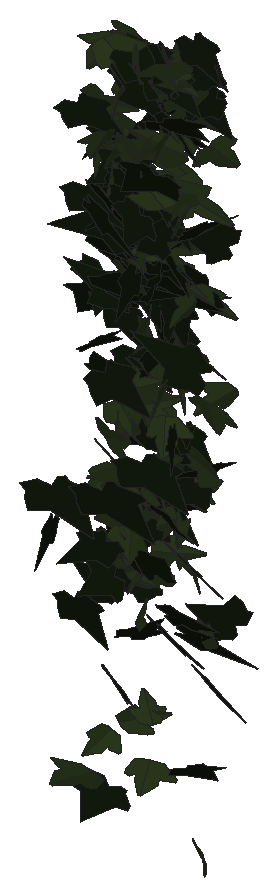
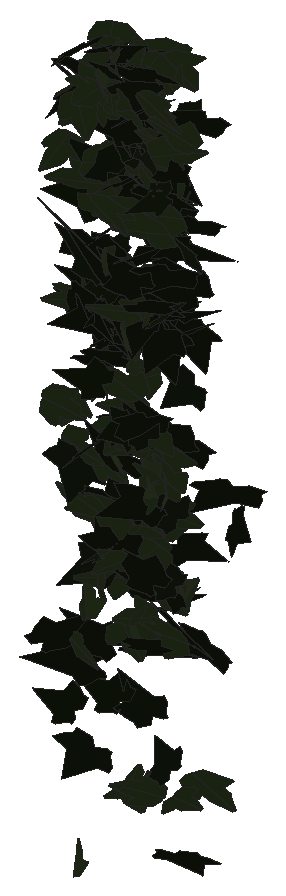
# SketchUp Ruby script. Lengths in millimetres.
U = 1.mm
M = Sketchup.active_model
def pt(a) = Geom::Point3d.new(a.map { |v| v * U })
def face(e, loops, mat)
  f = e.add_face(loops[0].map { |a| pt(a) })
  loops[1..].each { |l| e.add_face(l.map { |a| pt(a) }).erase! }
  f.material = f.back_material = mat if mat
  f
end
# faces: each face lists its corners as indices into pts; further lists are holes
def faces(e, pts, list, mat = nil) = list.each { |f| face(e, (f[0].is_a?(Array) ? f : [f]).map { |l| l.map { |i| pts[i] } }, mat) }
# xy, xz, yz: faces in a plane at the given z, y or x. An outline is a flat list of corners, or four numbers for a rectangle; further outlines are holes
def ring(l) = l.size == 4 ? [[l[0], l[1]], [l[2], l[1]], [l[2], l[3]], [l[0], l[3]]] : l.each_slice(2).to_a
def flat(e, list, mat, &to3) = list.each { |f| face(e, (f[0].is_a?(Array) ? f : [f]).map { |l| ring(l).map { |u, v| to3.(u, v) } }, mat) }
def xy(e, z, list, mat = nil) = flat(e, list, mat) { |x, y| [x, y, z] }
def xz(e, y, list, mat = nil) = flat(e, list, mat) { |x, z| [x, y, z] }
def yz(e, x, list, mat = nil) = flat(e, list, mat) { |y, z| [x, y, z] }
def lines(e, pts, list) = list.each { |a, b| e.add_line(pt(pts[a]), pt(pts[b])) }
# prism: a flat outline (further loops are holes) pulled along v
def prism(e, loops, v, mat = nil)
  f = face(e, loops, mat); d = Geom::Vector3d.new(v.map { |x| x * U })
  f.pushpull(f.normal.samedirection?(d) ? d.length : -d.length)
end
def box(e, o, s, mat = nil) = prism(e, [[o, [o[0] + s[0], o[1], o[2]], [o[0] + s[0], o[1] + s[1], o[2]], [o[0], o[1] + s[1], o[2]]]], [0, 0, s[2]], mat)
def at(x, y, z, deg = 0) = Geom::Transformation.translation(pt([x, y, z])) * Geom::Transformation.rotation(ORIGIN, Z_AXIS, deg.degrees)
def axes(o, x, y, z) = Geom::Transformation.new([*x, 0, *y, 0, *z, 0, *pt(o).to_a, 1])
def part(name) = M.definitions.add(name)
# library, detail: a bought-in or finely detailed component or shape, given as its bounding box
def library(name, o, s) = part(name).tap { |d| box(d.entities, o, s) }
def detail(e, o, s) = box(e.add_group.entities, o, s)
def put(e, d, t, mat = nil) = e.add_instance(d, t).tap { |i| i.material = mat if mat }
def group(e, t, mat = nil) = e.add_group.tap { |g| g.transformation = t; g.material = mat if mat }.entities
root = M.entities
M.materials.add("efeu1").color = [18, 25, 13]
M.materials.add("efeu2").color = [43, 57, 29]
c1 = part("ivyleaf_9")
p = [[39.1,54.8,31.7],[34.5,51.8,30.2],[-5.3,25.2,17.3],[-17.9,28.3,20.9],[-21.6,21.7,17],[-20.2,4.3,5.3],
  [-22.9,-0.3,2.5],[-17.1,-4,-0.6],[-2,-2.1,-1.2],[-0.7,-15.4,-10.1],[16.6,-22.3,-16.7],[21.1,-15.1,-12.5],
  [32.7,-10.7,-11],[46.1,-1.8,-6.6],[30.8,11.2,3.8]]
faces(c1.entities,p,[[0,1,2,3,4,5,6,7,8,9,10,11,12,13,14]],"efeu1")
c2 = part("ivyleaf_10")
p = [[0,12.8,-0.8],[-1.5,51.3,-10.9],[-4.9,51,-11.6],[-13.6,26.5,-7.3],[-13.2,15.9,-4.6],[-21.1,19.3,-7.2],
  [-29.5,16.3,-8.3],[-29.2,8.3,-6.2],[-19.7,-9.8,0.5],[-7.6,-13,4],[1,-12.2,5.8],[-0.4,51.1,-11.1],
  [-1.5,51.1,-10.9],[1,-12.4,5.9],[16.9,-12.4,3.5],[35.1,9.1,-5.1],[35,12.9,-6.1],[20.5,16.4,-4.9],
  [15.8,15,-3.8],[15.3,27.6,-7.1],[12.8,31.3,-7.8]]
faces(c2.entities,p,[[0,1,2,3,4,5,6,7,8,9,10],[11,12,0,13,14,15,16,17,18,19,20]],"efeu2")
put(root,c1,axes([2946.5,702.1,1430.8],[1.33754,-0.78365,-0.25205],[-0.30578,0.19446,-1.05258],[1.53656,0.72085,0.00994]))
put(root,c1,axes([2949.3,732.1,1125.1],[0.41508,-0.64574,-0.82159],[-0.25105,0.81557,-0.67602],[1.9729,0.23964,0.08683]))
put(root,c1,axes([2822.1,753.9,808],[-0.38061,0.24155,-0.98303],[1.27424,-0.71998,-0.31312],[-1.44495,-0.69854,-0.01719]))
put(root,c1,axes([2935.6,741.6,908.7],[-0.47588,-0.33732,-0.96585],[1.22364,0.72159,-0.41846],[1.51454,-0.68898,0.03461]))
put(root,c1,axes([2823.5,757.3,870.8],[-0.318,-0.64504,-0.79131],[0.5195,0.74442,-0.66445],[1.87224,-0.31611,0.04997]))
put(root,c1,axes([2974.1,780.6,1392.1],[-0.42556,-0.7327,0.45613],[-0.26926,-0.4337,-0.76602],[1.62038,-0.26449,-0.0075]))
put(root,c2,axes([2862.7,783.2,369.6],[-1.05005,-0.34553,0.61966],[-0.9573,-0.3631,-0.65033],[0.95229,-0.74602,0.02952]))
put(root,c1,axes([3000.5,781.7,1472.3],[0.68765,0.27193,-0.7739],[-1.19118,-0.45523,-0.45216],[-1.00913,0.72266,0.00638]))
put(root,c2,axes([3005.8,797.6,1091.6],[0.64746,-0.69061,0.64263],[0.46311,-0.59578,-0.76908],[1.73463,0.41684,-0.03454]))
put(root,c2,axes([2939.5,791.3,1504],[-0.96338,0.63955,-0.34988],[0.3885,-0.28456,-0.81548],[-1.33192,-0.54559,0.0152]))
put(root,c1,axes([2884.3,804.9,774.7],[-0.06144,-0.00892,-0.90166],[0.09196,-0.90096,0.00718],[-1.71366,-0.04803,0.03271]))
put(root,c2,axes([2883.4,802.4,1492.8],[-0.3913,-0.84361,0.13688],[-0.05405,-0.13396,-0.8683],[1.62566,-0.20752,0.00408]))
put(root,c1,axes([2969.8,796.5,945],[-0.29803,-0.55605,-0.80167],[0.77605,0.70032,-0.5654],[1.68688,-0.42042,0.11847]))
put(root,c1,axes([2941.8,807.7,1262],[-1.14315,0.31014,-0.74291],[1.21653,-0.37977,-0.67534],[-0.93146,-0.87663,0.02973]))
put(root,c2,axes([2917.2,802.9,909.6],[-0.86882,-0.86224,0.07932],[-0.05696,-0.0739,-0.97559],[1.64696,-0.45741,0.0081]))
put(root,c1,axes([2813.5,825.5,638.5],[-0.50737,-0.15268,-0.86245],[1.60954,0.18967,-0.29499],[0.43368,-0.88256,0.08581]))
put(root,c1,axes([2865.4,836.4,1351],[0.31051,-0.48763,0.92572],[0.80832,-0.82538,-0.50963],[1.81988,0.4498,0.06841]))
put(root,c1,axes([3044,831.6,1119.7],[-0.90393,-0.94187,-0.19726],[-0.16554,-0.17706,1.05485],[-1.82397,0.48285,0.00202]))
put(root,c1,axes([2872.5,841.2,694.4],[-0.6415,-0.54818,0.64582],[-0.65457,-0.54665,-0.6435],[1.47335,-0.48154,-0.0047]))
put(root,c1,axes([2828.8,815.6,1522.1],[0.05715,-0.35847,-0.79405],[0.35505,0.77874,-0.3445],[1.61964,-0.15806,0.10354]))
put(root,c2,axes([2971.9,827.2,1397.8],[0.86523,0.63733,0.38042],[-0.42946,-0.30632,0.78284],[1.34575,-0.50751,0.00524]))
put(root,c2,axes([3019.3,830.7,1389.7],[0.47653,-0.88746,0.00656],[0.00339,-0.00631,-0.9221],[1.68905,0.25039,0]))
put(root,c1,axes([2990.6,840.5,988.8],[-0.42942,-0.00366,-0.85863],[1.43073,-0.4298,-0.19572],[-0.7896,-0.7768,0.11233]))
put(root,c1,axes([2987.6,824.9,1333.3],[-1.1226,0.00585,-0.65301],[-1.24283,-0.01087,0.58976],[-0.00789,0.8799,0.01163]))
put(root,c2,axes([2900.3,838.1,806.8],[-1.15154,-0.78668,-0.1797],[-0.20357,-0.14443,0.99244],[-1.52222,0.61443,0.00322]))
put(root,c2,axes([2921.1,820.2,1053.7],[0.00615,-0.05009,-0.94639],[0.88673,0.82421,-0.04203],[1.57067,-0.46512,0.02743]))
put(root,c2,axes([2930.4,845.1,1570.4],[-0.98618,0.08628,0.76506],[1.36089,-0.28793,0.51677],[0.54319,0.87802,0.09429]))
put(root,c1,axes([2964,839.2,1573.9],[-1.49463,-0.31379,-0.39363],[-0.69423,-0.14797,0.84569],[-0.66026,0.8659,0.00187]))
put(root,c2,axes([2830,860.4,730.2],[-0.17259,-0.00456,-0.9556],[-0.1178,-0.95785,0.01044],[-1.81491,0.06261,0.0902]))
put(root,c1,axes([2906.7,840.4,1385.3],[-0.32136,-0.28061,-0.80655],[1.0862,0.5745,-0.31936],[1.20899,-0.59074,0.07253]))
put(root,c1,axes([2898.9,848,1400.9],[-0.97785,-0.11989,-0.67977],[1.27353,0.12147,-0.52719],[0.32243,-0.8434,0.0207]))
put(root,c2,axes([2984.5,840.1,1629.8],[-1.06364,-0.73144,-0.18088],[0.19582,0.14901,-0.92047],[1.42058,-0.5682,-0.00855]))
put(root,c2,axes([2904.6,837.7,1240.5],[-1.32865,0.47864,0.18463],[-0.29768,0.09836,-0.84641],[-0.92989,-0.71539,0.00716]))
put(root,c2,axes([2877.1,833.3,1633.5],[0.86639,0.81473,0.53404],[0.47429,0.47246,-0.93322],[-1.79233,0.51885,0.0112]))
put(root,c1,axes([2823,842.8,1360.1],[-0.01541,-0.61205,-0.66691],[0.56061,0.62885,-0.5807],[1.62899,-0.22221,0.19354]))
put(root,c2,axes([2924.8,849.2,1469.4],[-0.87338,-0.85692,0.21949],[-0.17095,-0.20085,-0.97194],[1.67484,-0.46736,0.01525]))
put(root,c2,axes([2863.5,855.2,1403.7],[-0.18078,0.57564,-0.62708],[-0.08598,-0.6335,-0.57469],[-1.61778,-0.03066,0.10062]))
put(root,c1,axes([2879,862.2,1308.3],[-0.31516,-0.43447,-0.95328],[-0.6344,-0.8931,0.46495],[-1.8902,0.37219,0.0029]))
put(root,c1,axes([2985.2,830.9,1537.9],[1.4509,0.56155,0.23401],[0.3381,0.15332,-0.94668],[-1.10736,0.78258,0.01756]))
put(root,c2,axes([2860.3,857.6,1625.5],[-0.84664,-0.74037,0.57588],[-0.26498,-0.57818,-0.85089],[1.76537,-0.44186,0.14846]))
put(root,c1,axes([2949,860.1,821.2],[1.64572,-0.49175,-0.28372],[0.50835,-0.10379,0.99395],[-0.95345,-0.90413,0.04021]))
put(root,c2,axes([2864.2,854.5,1589.3],[-0.79908,0.00825,0.84409],[1.55056,-0.24275,0.40762],[0.42043,0.91096,0.10098]))
put(root,c2,axes([2854.4,859.8,860.2],[0.64916,0.49909,-0.76047],[-0.79932,-0.63401,-0.60447],[-1.53561,0.541,-0.00684]))
put(root,c2,axes([2968.9,852.5,1501.7],[0.45157,-1.0565,0.06794],[0.03921,-0.06501,-1.0828],[2.0145,0.23809,0.00584]))
put(root,c2,axes([2886,832.1,1461.2],[-0.08461,-0.56041,-0.90692],[0.14712,0.90362,-0.56216],[2.02365,-0.08913,0.00295]))
put(root,c2,axes([2875.8,858.3,1554.7],[0.79106,-0.86728,0.37533],[0.36619,-0.32378,-0.96123],[1.76088,0.45695,0.03128]))
put(root,c2,axes([2988.5,846.2,1485.1],[0.01174,0.03823,0.95902],[-1.8257,-0.03073,0.0074],[0.05901,-0.95855,0.03801]))
put(root,c1,axes([2827.3,843.6,1303.9],[-0.10835,0.81888,0.22225],[0.02143,-0.222,0.82085],[1.61473,0.05789,0.00402]))
put(root,c2,axes([2935.7,845.7,1169.3],[0.12386,-0.91263,-0.40148],[0.08026,0.4045,-0.91265],[1.89587,0.0425,0.06487]))
put(root,c1,axes([2838.4,848.1,1180.8],[0.82597,0.43734,-0.60466],[-0.83165,-0.41808,-0.61603],[-1.15129,0.61577,0.0112]))
put(root,c1,axes([2968.3,848.1,1603.5],[0.0376,-0.57226,-0.67125],[0.1355,0.67026,-0.56932],[1.67329,-0.04142,0.06119]))
put(root,c2,axes([2990.5,854.1,1396.8],[-1.05575,-0.75141,0.09476],[-0.09596,-0.08056,-0.93396],[1.43821,-0.55696,0.00725]))
put(root,c2,axes([2976,844.7,1605.5],[-0.83826,-0.41984,-0.64128],[0.97998,0.3858,-0.60624],[1.0806,-0.67557,0.05233]))
put(root,c1,axes([2875.9,860,1185.6],[-1.02346,-0.71068,-0.22726],[-0.25807,-0.18238,0.8912],[-1.39638,0.55459,0.00186]))
put(root,c2,axes([2914.5,856.5,1626.2],[0.08211,0.82699,-0.28665],[-0.06771,-0.2851,-0.82788],[-1.66441,0.0524,0.01954]))
put(root,c2,axes([2888.9,859.1,765.2],[1.45175,-0.33876,0.22888],[0.39736,-0.09377,-0.83463],[0.66897,0.79085,-0.00093]))
put(root,c2,axes([3003.6,869.3,1210],[0.00855,-0.56231,0.70081],[0.15756,-0.69758,-0.56025],[1.70278,0.06737,0.04832]))
put(root,c2,axes([2821.7,864.4,1422.3],[-0.21788,0.62524,-0.58106],[0.06162,-0.58266,-0.63334],[-1.6233,-0.10603,0.05395]))
put(root,c2,axes([2963.2,858.9,985.5],[0.72711,0.86265,-0.25554],[-0.18918,-0.23546,-0.94345],[-1.70183,0.39474,-0.00431]))
put(root,c1,axes([2860.9,848.7,1191.7],[0.61464,0.00178,0.93752],[1.78424,-0.00819,-0.32293],[0.01364,0.99155,-0.00435]))
put(root,c1,axes([2910.6,853.2,1625.1],[0.33497,-0.63563,-0.80748],[0.52125,0.81862,-0.5847],[1.88506,-0.11341,0.30516]))
put(root,c1,axes([2940.7,871,1165.3],[-0.30707,0.10146,-0.94552],[1.60728,-0.42558,-0.18977],[-0.83199,-0.85961,-0.01765]))
put(root,c1,axes([2954.2,877.8,1613.4],[-0.32964,-0.53915,0.67346],[-0.34222,-0.64925,-0.56602],[1.60581,-0.24904,0.01762]))
put(root,c2,axes([2990.5,868.1,1560.3],[-0.78801,-0.84784,-0.28024],[-0.22024,-0.25534,0.94351],[-1.68514,0.42984,0.00773]))
put(root,c2,axes([2925.6,863.4,367],[1.0669,0.63253,-0.23032],[-0.30272,-0.16677,-0.84515],[-1.24487,0.58265,0.00813]))
put(root,c1,axes([2951.4,879.6,1270.2],[0.32272,-0.75576,0.7426],[0.26932,-0.72916,-0.77439],[1.99846,0.22031,-0.01556]))
put(root,c1,axes([2950.7,866.5,1521.3],[0.97395,-0.79217,0.0087],[0.00899,-0.0073,-0.94309],[1.50773,0.51176,0]))
put(root,c2,axes([2978.3,869.7,1068],[-0.33843,0.74198,-0.6107],[0.31377,-0.58831,-0.76277],[-1.80183,-0.24181,-0.01812]))
put(root,c2,axes([2835.5,871.9,389.2],[0.57962,0.47978,-0.64791],[-0.65027,-0.55052,-0.56826],[-1.38977,0.45768,-0.00433]))
put(root,c1,axes([2867.3,848.5,667.3],[-0.56179,0.58251,0.71709],[-0.74506,0.60302,-0.65099],[-1.59266,-0.48757,0.05159]))
put(root,c2,axes([2957,877.7,807.9],[-0.3015,0.25694,0.88052],[0.57235,-0.82962,0.29619],[1.64921,0.33489,0.05818]))
put(root,c2,axes([2915,858.5,1004.4],[-0.49123,0.83548,0.0138],[-0.01131,0.0126,-0.87444],[-1.59027,-0.25817,0.00196]))
put(root,c2,axes([2865.5,870.3,1473.1],[-0.52496,-0.08442,-0.81615],[-1.4399,-0.30706,0.28746],[-0.60435,0.80492,0.02406]))
put(root,c2,axes([2919,863.6,845.6],[1.03516,-0.68179,-0.08583],[0.10644,-0.06518,0.87216],[-1.30348,-0.54676,0.00305]))
put(root,c2,axes([2845.5,868.5,914.4],[-0.99136,0.18994,0.66639],[1.18633,-0.2357,0.55442],[0.57603,0.81231,0.00505]))
put(root,c2,axes([2969.2,876.4,1124],[0.02515,-0.14029,0.93823],[1.40708,-0.58644,-0.0981],[1.13135,0.73249,0.10115]))
put(root,c1,axes([3015.3,848.8,401.7],[1.0478,0.60789,0.21632],[0.26429,0.16607,-0.8201],[-1.19924,0.56773,0.00827]))
put(root,c2,axes([2872.5,858.7,715.5],[-1.15129,0.37549,-0.48891],[-0.78163,0.26536,0.71195],[0.87497,0.73113,-0.00731]))
put(root,c1,axes([2938.1,859.1,717.7],[0.43483,-0.3124,0.89181],[-1.0023,0.71971,0.38703],[-1.49322,-0.57406,-0.00009]))
put(root,c1,axes([2833.1,874.5,295.2],[-1.30661,-0.5213,-0.0395],[0.06964,0.01712,-0.86198],[0.99255,-0.68746,0.00848]))
put(root,c1,axes([2938.2,875.5,1403.8],[-0.16338,-0.92638,0.02959],[0.00476,-0.02995,-0.93033],[1.76398,-0.08572,0.00525]))
put(root,c2,axes([2823.8,863.4,1506],[-0.59125,-0.11348,0.79513],[1.47941,0.17213,0.32827],[-0.38481,0.83613,0.04034]))
put(root,c2,axes([2971.5,875.5,915.6],[-0.24835,-0.67748,0.49323],[-0.20405,-0.48157,-0.68983],[1.58178,-0.16849,-0.01155]))
put(root,c1,axes([2949.3,850.7,1116.2],[0.01199,-0.07492,-0.88045],[-0.63621,0.81483,-0.07173],[1.55674,0.33358,-0.02253]))
put(root,c1,axes([2805.6,870.5,1257.2],[1.61537,0.03663,-0.41211],[0.77316,0.10441,0.84596],[0.14918,-0.93773,0.07809]))
put(root,c1,axes([2824.9,850,1086.1],[0.68232,0.56861,0.52911],[0.50558,0.45785,-0.67202],[-1.38908,0.44594,0.01531]))
put(root,c1,axes([2840.1,874.2,744],[0.01033,-0.03981,-0.82611],[1.57408,0.00006,0.00543],[-0.00038,-0.82613,0.03981]))
put(root,c2,axes([2928.5,855.5,1009.5],[-0.19949,-0.27405,0.82991],[0.46446,0.79343,0.29283],[-1.59721,0.26496,-0.0185]))
put(root,c1,axes([2817.3,885.6,1189.8],[-0.44104,-0.86592,0.27709],[-0.08526,-0.27473,-0.896],[1.72824,-0.23453,0.02651]))
put(root,c1,axes([2862.1,885.8,1391.8],[-0.8509,-0.43393,0.52991],[-0.60564,-0.42876,-0.61959],[1.15428,-0.54485,0.06554]))
put(root,c1,axes([3012.3,852.1,1343.9],[-0.04025,0.76391,-0.54859],[-0.09767,0.54697,0.76363],[1.78726,0.04709,0.02938]))
put(root,c2,axes([2894.7,876.6,829.9],[1.03352,0.56281,-0.43949],[-0.58024,-0.31655,-0.78208],[-1.22894,0.62277,-0.00035]))
put(root,c2,axes([2941.6,885.6,1610.6],[0.08457,-0.25729,0.94876],[1.32946,-0.65996,-0.21169],[1.31635,0.68306,0.15284]))
put(root,c1,axes([2931.4,876.8,1204.8],[-1.18885,-0.44863,-0.62446],[0.95688,0.37041,-0.76905],[1.10719,-0.80184,-0.00587]))
put(root,c1,axes([2827.3,885.3,875.9],[1.16834,-0.26296,-0.61355],[1.05525,-0.26329,0.6676],[-0.70742,-0.82703,-0.01745]))
put(root,c2,axes([2912.3,859.3,626.1],[0.22078,-0.1999,0.80285],[-0.69447,0.71524,0.23081],[-1.41323,-0.3827,0.012]))
put(root,c1,axes([2843.3,881.2,1454.4],[-0.34875,0.46361,-0.69577],[0.41557,-0.66103,-0.49797],[-1.536,-0.28411,0.02325]))
put(root,c1,axes([2908,887.9,1608.3],[-1.51562,-0.51494,-0.12466],[0.20771,0.06079,-0.9483],[0.98672,-0.80376,0.00814]))
put(root,c1,axes([2939.6,881.5,1206.5],[0.65927,-0.25474,0.81027],[1.30373,-0.43358,-0.42917],[0.95574,0.76717,0.02651]))
put(root,c2,axes([2949.1,887.7,1450.9],[-0.65509,-0.26523,0.88729],[-1.26958,-0.58559,-0.43382],[1.22256,-0.75023,0.02493]))
put(root,c1,axes([2934.7,862.9,1221.7],[-0.71976,0.2782,-0.85775],[-1.41034,0.4341,0.46752],[0.97787,0.83085,0.04294]))
put(root,c1,axes([2930.3,887.1,859],[-1.38206,-0.26803,-0.29018],[0.51214,0.10891,-0.77402],[0.55038,-0.77439,-0.00842]))
put(root,c1,axes([2919.1,875.8,1469.8],[1.47502,-0.30093,-0.2517],[-0.42011,0.12624,-0.83061],[0.61726,0.80503,0.03616]))
put(root,c2,axes([2874.9,879.1,819.4],[-0.88826,-0.07216,-0.68645],[1.31361,-0.04209,-0.46485],[0.01063,-0.82902,0.08335]))
put(root,c1,axes([2888.2,890.2,780.6],[-1.40912,-0.49075,-0.31249],[0.50169,0.1679,-0.88825],[0.9871,-0.7859,0.00537]))
put(root,c2,axes([2938.2,894.8,954.8],[0.65091,-0.6783,0.58779],[0.44358,-0.54032,-0.75913],[1.6496,0.41294,-0.0278]))
put(root,c2,axes([2980.5,878.9,1389.4],[0.72615,0.15398,0.97579],[1.76952,0.2975,-0.41049],[-0.63532,1.00461,-0.028]))
put(root,c1,axes([2851.8,884.6,1140.9],[0.35514,-0.78798,-0.33888],[-0.12406,0.33277,-0.80968],[1.62776,0.19728,0.01223]))
put(root,c1,axes([2934.3,882.1,923.2],[-0.79507,0.36828,0.74908],[1.00411,-0.53262,0.55609],[1.23107,0.67228,0.03021]))
put(root,c2,axes([3036.3,870.1,924.7],[0.05561,0.07757,-1.0189],[-1.30754,0.75604,0.03785],[1.43963,0.68368,0.07374]))
put(root,c1,axes([2875.4,883.6,1576.1],[1.68359,-0.46342,0.30091],[0.51982,-0.12703,-0.99855],[0.91414,0.92572,0.01362]))
put(root,c2,axes([2909.2,887.8,1108],[-1.06619,0.64858,0.27437],[0.34156,-0.20754,0.85703],[1.29604,0.58826,-0.00015]))
put(root,c2,axes([2850.7,886.9,1416.7],[-1.21284,-0.24393,0.44855],[0.88624,0.01659,0.67059],[-0.39859,0.77912,0.12616]))
put(root,c1,axes([2918.7,878.4,1485],[-1.01724,0.90076,-0.00372],[0.00016,-0.00428,-1.0474],[-1.71434,-0.53449,0.00211]))
put(root,c1,axes([2962.4,882,751],[1.71636,-0.44317,-0.15553],[-0.24926,0.08607,-1.00465],[0.85841,0.91108,0.01925]))
put(root,c2,axes([3008.8,892.6,217.4],[-0.80589,0.50367,0.49473],[0.60433,-0.37938,0.65802],[1.20009,0.52927,0.00087]))
put(root,c2,axes([2912.8,885.4,1061.6],[-0.93283,-0.18346,0.74154],[1.31858,0.26435,0.52334],[-0.61238,0.84867,-0.00272]))
put(root,c1,axes([2976.9,902.4,1105.4],[-1.31843,-0.27828,0.53933],[-0.9198,-0.2421,-0.74568],[0.69863,-0.8439,0.03607]))
put(root,c1,axes([2830.9,894.4,1004.9],[-0.50956,-0.05716,0.88124],[1.30659,-0.59269,0.17013],[1.05717,0.70497,0.21449]))
put(root,c1,axes([2886.4,892.6,1421.7],[-1.6369,0.45628,-0.14401],[0.23326,-0.07625,-0.97357],[-0.88024,-0.86871,0.00981]))
put(root,c1,axes([3029.5,895.2,1568.3],[-1.43668,0.2554,-0.26246],[0.45178,-0.11666,-0.79624],[-0.53075,-0.79065,0.0327]))
put(root,c1,axes([2980.7,901.1,872.2],[-1.84931,-0.14808,-0.00848],[0.01604,0.001,-0.9829],[0.28183,-0.97172,0.00028]))
put(root,c1,axes([2863.3,889.7,1564.5],[0.61591,-0.67478,-0.53496],[-0.08006,0.55842,-0.72982],[1.63691,0.28121,0.16559]))
put(root,c2,axes([2882.2,909.6,680.8],[0.24667,-0.45824,0.7792],[0.34428,-0.7581,-0.47592],[1.68562,0.2219,-0.01682]))
put(root,c1,axes([2929,894.6,1344.6],[0.54125,-0.79283,-0.3611],[-0.24753,0.33696,-0.84226],[1.63947,0.31262,-0.00795]))
put(root,c2,axes([2869.3,891,807.3],[-1.54261,0.0469,-0.42897],[0.81639,-0.01189,-0.81181],[-0.08949,-0.91697,-0.01142]))
put(root,c2,axes([2819.7,898.9,676.9],[-0.27434,-0.00685,-0.98136],[1.73286,-0.37106,-0.13115],[-0.69696,-0.91987,0.06021]))
put(root,c1,axes([2943,898.1,625.4],[1.22062,0.09368,-0.50962],[0.95547,0.08838,0.64805],[0.24409,-0.81439,0.01171]))
put(root,c1,axes([2911.7,896.6,1281.7],[-0.92234,-0.68658,0.17349],[0.18367,0.14423,0.84038],[-1.3352,0.49412,-0.00424]))
put(root,c1,axes([2818.2,911.8,462.7],[0.99349,-0.30648,-0.677],[1.11974,-0.33499,0.6053],[-0.86403,-0.78652,0.006]))
put(root,c2,axes([2850.2,908.9,938.7],[-0.38265,0.00906,0.79456],[1.15977,-0.52423,0.16018],[0.97055,0.63002,0.12185]))
put(root,c2,axes([2968.8,885.4,779.2],[0.74416,-0.30598,0.88595],[-1.21353,0.61676,0.49442],[-1.30748,-0.74659,0.04535]))
put(root,c1,axes([2865.4,896.6,1188.7],[0.84393,0.65671,-0.6723],[-0.71388,-0.55794,-0.7924],[-1.64003,0.5808,-0.00104]))
put(root,c2,axes([2865.4,912.9,1226.6],[-0.2559,0.2921,-0.82646],[0.61969,-0.75965,-0.32146],[-1.5489,-0.35218,0.00793]))
put(root,c2,axes([2966.6,914.5,1607],[-0.17579,-0.50742,0.7116],[-0.32379,-0.69144,-0.51512],[1.63155,-0.19189,-0.02556]))
put(root,c1,axes([2971.7,900.5,956.3],[0.56443,-0.72446,-0.39418],[-0.27867,0.36598,-0.78281],[1.54474,0.33073,0.00281]))
put(root,c1,axes([3009.3,885.2,911.1],[0.66215,0.87464,0.18615],[0.1183,0.17561,-0.94127],[-1.69778,0.35335,0.00702]))
put(root,c2,axes([3022.5,897.5,1018.5],[-1.63387,0.2685,0.05403],[-0.09937,0.01407,-0.89949],[-0.51168,-0.86007,0.00216]))
put(root,c2,axes([2880.5,886.4,686.6],[0.2495,-0.20385,0.83717],[0.27151,0.84025,0.18226],[-1.61722,0.10962,0.15975]))
put(root,c2,axes([2824.6,915.3,925.4],[-0.0719,0.39473,-0.77688],[0.16236,-0.7722,-0.3965],[-1.6505,-0.09316,-0.00516]))
put(root,c2,axes([2895.6,895.8,1380.8],[-0.83531,-0.16426,-0.72473],[1.30188,0.23956,-0.46855],[0.55258,-0.8127,0.00837]))
put(root,c1,axes([2984,910.5,1603.2],[-1.32454,-0.43216,-0.32261],[0.52812,0.16466,-0.81919],[0.88009,-0.74921,0.00605]))
put(root,c1,axes([2899.3,900.4,1517],[1.09046,-0.13827,0.57344],[1.06489,-0.1257,-0.58937],[0.35543,0.80082,0.0065]))
put(root,c2,axes([2930.3,890.1,739.3],[-0.19965,-0.05217,-0.90399],[1.34197,0.56623,-0.1145],[1.08119,-0.71244,-0.02481]))
put(root,c1,axes([2845.1,911.3,1432.4],[-1.46445,-0.31414,-0.21104],[0.36535,0.08809,-0.83108],[0.62071,-0.793,-0.00872]))
put(root,c1,axes([2937.4,909.8,1169.4],[-0.89031,-0.08667,-0.72352],[1.37175,0.07151,-0.47458],[0.20412,-0.85861,0.03351]))
put(root,c2,axes([2994.8,896.5,1537.2],[-1.13248,-0.60988,-0.48951],[0.61656,0.3676,-0.8518],[1.35464,-0.67717,-0.02153]))
put(root,c1,axes([3052.6,895.2,1317.6],[-1.04039,0.67911,0.44936],[-0.51672,0.35826,-0.87171],[-1.46113,-0.61025,-0.01169]))
put(root,c2,axes([2963.5,890.7,1059.6],[0.12618,0.49334,-0.68548],[0.18937,0.67824,0.49775],[1.59616,-0.11946,-0.00487]))
put(root,c2,axes([2942.1,917.4,732.1],[0.08908,-0.12777,0.80813],[1.21808,-0.49853,-0.11589],[0.97002,0.63775,0.07132]))
put(root,c2,axes([2927.1,907.2,858.2],[-1.1475,0.22787,-0.73093],[1.31132,-0.2442,-0.64448],[-0.63538,-0.91551,-0.01002]))
put(root,c1,axes([2923.8,906.3,1254.2],[1.50371,-0.59008,-0.12677],[-0.1872,0.08016,-0.98611],[1.1333,0.79618,0.00532]))
put(root,c2,axes([2864.1,902.9,1018],[-1.51424,-0.16177,-0.49221],[0.91227,0.11255,-0.81181],[0.37429,-0.92878,-0.01265]))
put(root,c1,axes([2933.1,893.1,1212],[0.25838,-0.00107,-0.81488],[-0.62918,0.75501,-0.05606],[1.41753,0.33531,0.12365]))
put(root,c2,axes([2931.2,911.1,1293.6],[-0.08367,-0.89604,0.03976],[-0.00527,-0.03967,-0.89712],[1.70702,-0.04404,-0.00082]))
put(root,c1,axes([2920.3,914.1,1164.9],[0.11686,-0.83782,-0.22154],[-0.08178,0.21888,-0.83966],[1.64731,0.0703,-0.02597]))
put(root,c1,axes([2992.6,905.9,1557.4],[0.3824,-0.75038,-0.60078],[-0.28842,0.58136,-0.7768],[1.80657,0.25165,0.00315]))
put(root,c1,axes([2823.7,906.4,1303.7],[-0.25508,-0.63271,-0.7364],[0.35089,0.71327,-0.64639],[1.81415,-0.22692,0.02148]))
put(root,c1,axes([2879.9,920.1,653.2],[-1.08713,-0.14749,0.61094],[-1.10391,-0.19418,-0.58919],[0.46058,-0.81353,0.02987]))
put(root,c1,axes([2872.6,911.3,763.6],[-0.48784,0.30771,0.8247],[1.02908,-0.62274,0.40041],[1.32192,0.59835,-0.00737]))
put(root,c2,axes([2833.6,912.5,943.8],[1.32582,-0.03017,0.52696],[1.00076,-0.03618,-0.6972],[0.08732,0.87274,-0.01069]))
put(root,c1,axes([2911.9,913.2,806.6],[1.45287,0.25651,0.13275],[-0.23882,-0.04332,0.80533],[0.49511,-0.77363,-0.00108]))
put(root,c1,axes([2854.9,920.3,1018.4],[1.1614,-0.1825,-0.46421],[0.84413,-0.13705,0.63693],[-0.43432,-0.75438,-0.00341]))
put(root,c2,axes([2906.1,907.1,1261.9],[-0.61455,-0.16237,0.88721],[1.552,0.3501,0.36087],[-0.73347,0.87684,0.02021]))
put(root,c1,axes([2978.4,912,1639.1],[0.44228,-0.8098,-0.40261],[-0.11405,0.40098,-0.84113],[1.7174,0.23517,0.04782]))
put(root,c2,axes([2986.1,911.3,1202.6],[-0.89964,-0.01443,-0.69725],[1.32117,-0.09048,-0.46875],[-0.12723,-0.8375,0.06266]))
put(root,c2,axes([2892.8,909.8,988.8],[1.13128,0.27666,0.48443],[0.84075,0.19886,-0.65562],[-0.64837,0.74057,-0.00492]))
put(root,c2,axes([2897.6,916.4,672.5],[-1.12873,-0.57129,0.255],[-0.35065,-0.1763,-0.82347],[1.13787,-0.62103,-0.00081]))
put(root,c2,axes([2815.4,912.4,1402.6],[-0.58201,0.00048,-0.79574],[1.50815,-0.07754,-0.30458],[-0.13807,-0.84894,0.02737]))
put(root,c2,axes([3008.8,906.7,610.6],[-0.39074,0.1267,0.79196],[-1.44441,0.23367,-0.23413],[-0.49361,-0.78406,0.0582]))
put(root,c1,axes([2812.9,921.3,1241.5],[0.45879,-0.84777,-0.03134],[-0.01094,0.03095,-0.88138],[1.61455,0.24111,0.00293]))
put(root,c1,axes([2964.6,909.1,1308.4],[0.55186,0.76052,-0.38598],[-0.27122,-0.35874,-0.81391],[-1.60035,0.32305,0.00484]))
put(root,c2,axes([2965.1,913,855.4],[0.9307,-0.02601,-0.62997],[1.19775,-0.02843,0.4897],[-0.0731,-0.79699,0.00309]))
put(root,c1,axes([2990.5,928.1,510.8],[0.70421,-0.60724,0.58866],[0.52712,-0.5201,-0.71061],[1.52084,0.46144,-0.02628]))
put(root,c1,axes([2899.1,924.8,1471.8],[0.93344,-0.67686,0.32212],[0.35106,-0.26412,-0.83586],[1.38277,0.52397,-0.00523]))
put(root,c2,axes([2985.6,918.7,1542.1],[-0.87912,-0.9782,0.03968],[-0.03144,-0.03608,-1.08178],[1.86298,-0.46221,0.00047]))
put(root,c1,axes([2966.5,913.2,591.4],[1.48322,-0.17074,0.48973],[0.91877,-0.0843,-0.79762],[0.3608,0.91656,0.01787]))
put(root,c1,axes([2924.2,919.9,804.8],[0.62169,-0.691,-0.20454],[-0.16372,0.18558,-0.76432],[1.3617,0.33779,0.00149]))
put(root,c2,axes([2957.3,929.5,690.3],[-1.07714,0.35181,0.69168],[0.91605,-0.51238,0.65445],[1.1585,0.73226,0.12562]))
put(root,c1,axes([2799.4,926.8,786.7],[0.76457,-0.55209,0.36953],[0.43712,-0.2898,-0.68265],[1.18643,0.46255,0.01337]))
put(root,c1,axes([2887,911.5,1220.8],[1.32505,0.5089,-0.45215],[-0.72232,-0.24674,-0.86211],[-1.07557,0.79265,0.02193]))
put(root,c1,axes([2848.7,919.6,549.3],[1.11395,0.57496,0.19386],[-0.26919,-0.13264,0.82045],[1.12298,-0.60213,0.00437]))
put(root,c2,axes([2856,906.6,404.6],[-0.22582,-0.32298,0.86052],[0.59968,0.80079,0.34401],[-1.6433,0.33661,0.00729]))
put(root,c2,axes([2922.2,935.2,1562.7],[-0.16425,-0.58021,0.63508],[0.31383,-0.63759,-0.5601],[1.60681,0.06522,0.17431]))
put(root,c1,axes([2949.6,916,1274],[0.60789,0.87127,0.13479],[-0.13219,-0.11805,0.92765],[1.67271,-0.32596,0.02432]))
put(root,c2,axes([3018.1,937.8,1026.4],[-0.3332,-0.56918,0.78491],[-0.2336,-0.77818,-0.59168],[1.83043,-0.20292,0.06737]))
put(root,c2,axes([2951.7,937.3,1459.7],[0.11479,0.2385,-0.84343],[-0.81512,-0.72961,-0.23694],[-1.45545,0.42742,0.06618]))
put(root,c1,axes([2996.1,917.4,1213.6],[0.18884,0.04757,-0.94181],[-1.78038,-0.11458,-0.10434],[-0.22655,0.94007,0.03494]))
put(root,c1,axes([2854,915.7,901.6],[1.46739,0.0822,0.23734],[0.44478,0.04598,-0.77512],[-0.17515,0.8054,0.02003]))
put(root,c1,axes([2825,916.5,1206.3],[1.58287,-0.00458,-0.48617],[-0.9253,-0.00139,-0.83169],[0.00618,0.96336,-0.00351]))
put(root,c2,axes([2883.9,919.2,417.1],[0.42828,0.77662,-0.08698],[-0.00318,0.09099,0.80812],[1.4873,-0.22344,0.02677]))
put(root,c1,axes([2898.1,935.5,563],[0.61372,-0.57829,0.62565],[0.67744,-0.51634,-0.66071],[1.47318,0.47835,0.04319]))
put(root,c2,axes([2902.9,915.7,790.6],[0.56442,0.48312,0.58567],[0.57045,0.5032,-0.56685],[-1.32758,0.42161,0.00543]))
put(root,c1,axes([2833.4,935.7,785.1],[0.30148,-0.24023,0.87138],[0.97775,-0.70395,-0.28746],[1.41541,0.53745,0.01297]))
put(root,c2,axes([2872.9,934.7,1573],[0.8835,-0.2594,0.66136],[1.11373,-0.30832,-0.53168],[0.7666,0.74688,0.01022]))
put(root,c2,axes([3011.5,915.9,1465.4],[-0.68693,-0.74129,-0.69095],[0.74297,0.57515,-0.82098],[1.77981,-0.5262,0.07604]))
put(root,c2,axes([2847.6,914.4,915.2],[0.35218,-0.35823,0.70226],[-0.53847,0.64311,0.40261],[-1.40044,-0.33737,0.0218]))
put(root,c1,axes([2942.9,911.8,1183.8],[0.91338,0.31849,0.65235],[1.02312,0.36962,-0.57594],[-0.92849,0.7206,0.00709]))
put(root,c2,axes([2828.8,924.5,1376],[0.68576,0.11434,0.88818],[1.62043,0.25294,-0.37797],[-0.52814,0.92451,-0.00643]))
put(root,c2,axes([2885.8,930.5,1190.9],[0.28224,-0.84263,0.03176],[0.01028,-0.03129,-0.85558],[1.6048,0.14839,-0.0001]))
put(root,c1,axes([2855.1,922.4,1049.3],[-0.07486,-0.56855,-0.72009],[0.07101,0.71917,-0.56986],[1.74473,-0.05367,-0.0077]))
put(root,c1,axes([3029.3,942,620.1],[0.00739,0.08176,1.01596],[-1.56863,-0.59744,0.05123],[1.1412,-0.82174,0.06384]))
put(root,c2,axes([2870,917.6,1219.6],[0.02233,-0.09017,-0.96091],[1.68709,0.38104,-0.02493],[0.7264,-0.88221,0.08744]))
put(root,c2,axes([2947.3,928.5,1580.6],[-1.40663,0.23851,-0.3664],[0.6271,-0.16911,-0.77474],[-0.54687,-0.8074,0.05403]))
put(root,c2,axes([2933.9,930.7,1600.9],[0.57021,-0.81599,-0.04519],[-0.02289,0.04372,-0.86925],[1.55521,0.29983,0.00377]))
put(root,c1,axes([2861.4,933.2,1279.2],[1.33337,0.05502,-0.37636],[0.7136,0.0327,0.70274],[0.12169,-0.79461,0.00286]))
put(root,c1,axes([2916.9,939.6,1459],[0.31756,-0.43211,0.71695],[0.86126,-0.56846,-0.44793],[1.3403,0.46767,0.11797]))
put(root,c1,axes([2930,936.5,1088.7],[0.91579,-0.55843,0.45126],[0.59301,-0.32699,-0.73689],[1.23105,0.57293,0.01927]))
put(root,c2,axes([2943,929.1,1391.5],[1.44033,-0.1709,-0.51183],[-0.92563,0.16585,-0.77451],[0.44484,0.89844,0.04562]))
put(root,c1,axes([2848.7,943.7,1254.7],[-1.21282,-0.47299,0.3462],[-0.48084,-0.2398,-0.79267],[1.00661,-0.68443,0.03847]))
put(root,c1,axes([2814.8,928.3,1444.1],[1.23052,-0.50733,-0.14909],[-0.17991,0.1208,-0.82105],[0.99017,0.65243,0.03609]))
put(root,c1,axes([2898.5,911.5,1012.4],[0.36549,0.32882,0.76951],[0.69403,0.67773,-0.38061],[-1.43347,0.41197,0.01193]))
put(root,c2,axes([2847.9,923.9,1594.3],[0.76871,-0.29481,-0.75471],[-1.16501,0.44146,-0.50005],[1.0103,0.73337,-0.00238]))
